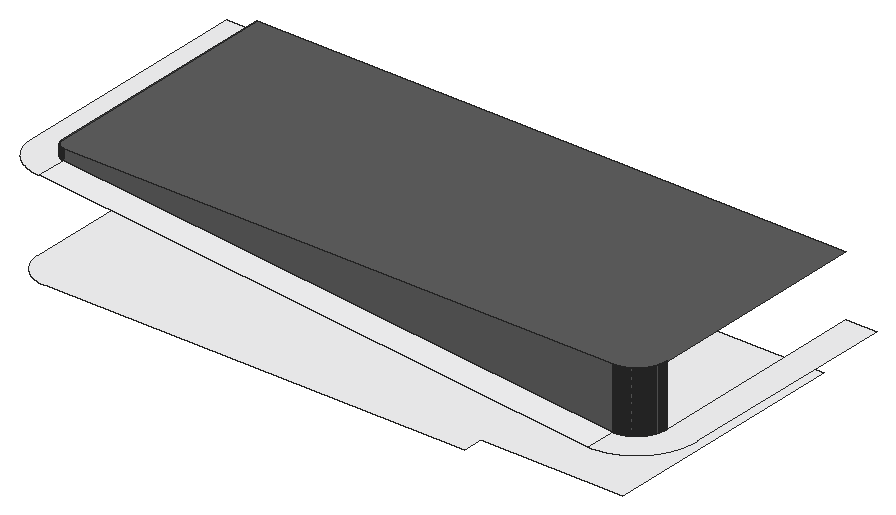
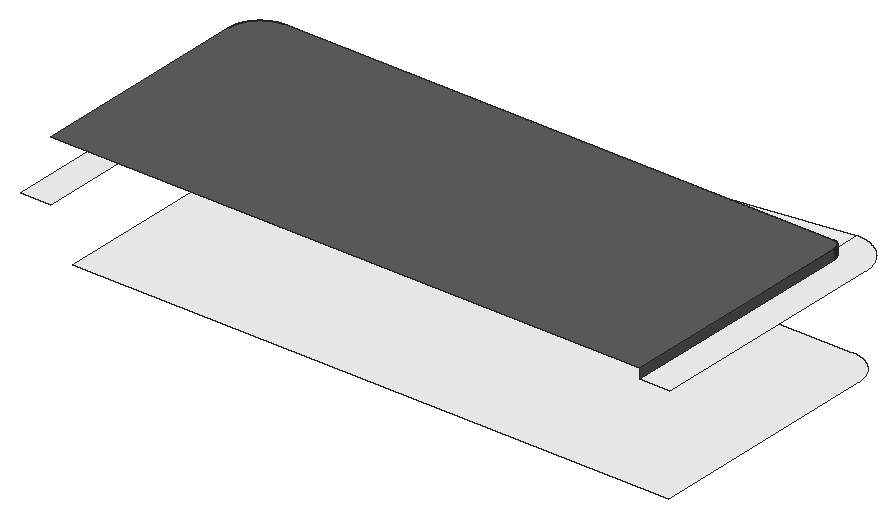
# SketchUp Ruby script. Lengths in inches.
U = 1.inch
M = Sketchup.active_model
def pt(a) = Geom::Point3d.new(a.map { |v| v * U })
def face(e, loops, mat)
  f = e.add_face(loops[0].map { |a| pt(a) })
  loops[1..].each { |l| e.add_face(l.map { |a| pt(a) }).erase! }
  f.material = f.back_material = mat if mat
  f
end
# faces: each face lists its corners as indices into pts; further lists are holes
def faces(e, pts, list, mat = nil) = list.each { |f| face(e, (f[0].is_a?(Array) ? f : [f]).map { |l| l.map { |i| pts[i] } }, mat) }
# xy, xz, yz: faces in a plane at the given z, y or x. An outline is a flat list of corners, or four numbers for a rectangle; further outlines are holes
def ring(l) = l.size == 4 ? [[l[0], l[1]], [l[2], l[1]], [l[2], l[3]], [l[0], l[3]]] : l.each_slice(2).to_a
def flat(e, list, mat, &to3) = list.each { |f| face(e, (f[0].is_a?(Array) ? f : [f]).map { |l| ring(l).map { |u, v| to3.(u, v) } }, mat) }
def xy(e, z, list, mat = nil) = flat(e, list, mat) { |x, y| [x, y, z] }
def xz(e, y, list, mat = nil) = flat(e, list, mat) { |x, z| [x, y, z] }
def yz(e, x, list, mat = nil) = flat(e, list, mat) { |y, z| [x, y, z] }
def lines(e, pts, list) = list.each { |a, b| e.add_line(pt(pts[a]), pt(pts[b])) }
# prism: a flat outline (further loops are holes) pulled along v
def prism(e, loops, v, mat = nil)
  f = face(e, loops, mat); d = Geom::Vector3d.new(v.map { |x| x * U })
  f.pushpull(f.normal.samedirection?(d) ? d.length : -d.length)
end
def box(e, o, s, mat = nil) = prism(e, [[o, [o[0] + s[0], o[1], o[2]], [o[0] + s[0], o[1] + s[1], o[2]], [o[0], o[1] + s[1], o[2]]]], [0, 0, s[2]], mat)
def at(x, y, z, deg = 0) = Geom::Transformation.translation(pt([x, y, z])) * Geom::Transformation.rotation(ORIGIN, Z_AXIS, deg.degrees)
def axes(o, x, y, z) = Geom::Transformation.new([*x, 0, *y, 0, *z, 0, *pt(o).to_a, 1])
def part(name) = M.definitions.add(name)
# library, detail: a bought-in or finely detailed component or shape, given as its bounding box
def library(name, o, s) = part(name).tap { |d| box(d.entities, o, s) }
def detail(e, o, s) = box(e.add_group.entities, o, s)
def put(e, d, t, mat = nil) = e.add_instance(d, t).tap { |i| i.material = mat if mat }
def group(e, t, mat = nil) = e.add_group.tap { |g| g.transformation = t; g.material = mat if mat }.entities
root = M.entities
M.materials.add("1421 AP 8232 ELEGANT GREY").color = [96, 96, 96]
M.materials.add("[Quartz Light Grey]").color = [251, 251, 252]
xy(root,234,[[47.74,189,47.61,189.01,47.48,189.01,47.22,189.03,47.08,189.04,46.95,189.05,46.69,189.09,46.57,189.1,46.4375,189.125,46.31,189.14,46.18,189.17,46.05,189.19,45.79,189.25,45.67,189.28,45.41,189.34,45.29,189.375,45.16,189.41,45.03,189.45,44.79,189.53,44.66,189.57,44.54,189.62,44.42,189.66,44.29,189.71,44.17,189.76,44.05,189.8125,43.93,189.86,43.8125,189.92,43.69,189.97,43.58,190.03,43.34,190.15,43.23,190.21,43.11,190.28,43,190.34,42.89,190.41,42.78,190.47,42.66,190.54,42.55,190.61,42.44,190.69,42.34,190.76,42.23,190.83,42.12,190.91,42.02,190.99,41.91,191.07,41.71,191.23,41.61,191.3125,41.51,191.4,41.41,191.48,41.21,191.66,41.12,191.75,41.02,191.84,40.84,192.02,40.75,192.12,40.66,192.21,40.48,192.41,40.4,192.51,40.3125,192.61,40.23,192.71,40.07,192.91,39.99,193.02,39.91,193.12,39.83,193.23,39.76,193.34,39.69,193.44,39.61,193.55,39.54,193.66,39.47,193.78,39.41,193.89,39.34,194,39.28,194.11,39.21,194.23,39.15,194.34,39.03,194.58,38.97,194.69,38.92,194.8125,38.86,194.93,38.8125,195.05,38.76,195.17,38.71,195.29,38.66,195.42,38.62,195.54,38.57,195.66,38.53,195.79,38.45,196.03,38.41,196.16,38.375,196.29,38.34,196.41,38.28,196.67,38.25,196.79,38.19,197.05,38.17,197.18,38.14,197.31,38.125,197.4375,38.1,197.57,38.09,197.69,38.05,197.95,38.04,198.08,38.03,198.22,38.01,198.48,38.01,198.61,38,198.74,38,269,214,269,214,195,172,195,172,189]],"[Quartz Light Grey]")
xy(root,249,[[210,187,210.24,187,210.47,187.01,210.71,187.01,210.94,187.02,211.18,187.04,211.41,187.06,211.65,187.08,211.88,187.1,212.12,187.125,212.35,187.15,212.58,187.1875,212.82,187.22,213.28,187.3,213.51,187.35,213.74,187.39,213.97,187.44,214.2,187.5,214.43,187.55,214.66,187.61,214.89,187.68,215.11,187.74,215.34,187.81,215.5625,187.88,215.79,187.96,216.01,188.03,216.23,188.11,216.45,188.2,216.67,188.28,217.11,188.46,217.32,188.56,217.54,188.65,217.75,188.75,217.96,188.86,218.17,188.96,218.59,189.18,218.8,189.3,219,189.41,219.4,189.65,219.61,189.78,219.8,189.9,220,190.03,220.2,190.17,220.39,190.3,220.58,190.4375,220.77,190.58,220.96,190.72,221.14,190.86,221.33,191.01,221.51,191.16,221.69,191.3125,221.87,191.47,222.04,191.625,222.22,191.78,222.39,191.94,222.56,192.11,222.73,192.27,222.89,192.44,223.06,192.61,223.22,192.78,223.375,192.96,223.53,193.13,223.6875,193.31,223.84,193.49,223.99,193.67,224.14,193.86,224.28,194.04,224.42,194.23,224.5625,194.42,224.7,194.61,224.83,194.8,224.97,195,225.1,195.2,225.22,195.39,225.35,195.6,225.59,196,225.7,196.2,225.82,196.41,226.04,196.83,226.14,197.04,226.25,197.25,226.35,197.46,226.44,197.68,226.54,197.89,226.72,198.33,226.8,198.55,226.89,198.77,226.97,198.99,227.04,199.21,227.12,199.4375,227.19,199.66,227.26,199.89,227.32,200.11,227.39,200.34,227.45,200.57,227.5,200.8,227.56,201.03,227.61,201.26,227.65,201.49,227.7,201.72,227.78,202.18,227.8125,202.42,227.85,202.65,227.875,202.88,227.9,203.12,227.92,203.35,227.94,203.59,227.96,203.82,227.98,204.06,227.99,204.29,227.99,204.53,228,204.76,228,271,219,271,219,204.76,218.99,204.65,218.99,204.53,218.97,204.29,218.96,204.18,218.95,204.06,218.9375,203.94,218.92,203.83,218.91,203.71,218.89,203.59,218.87,203.48,218.83,203.24,218.8,203.13,218.78,203.01,218.75,202.9,218.72,202.78,218.66,202.56,218.63,202.44,218.6,202.33,218.48,202,218.44,201.88,218.36,201.66,218.31,201.56,218.27,201.45,218.17,201.23,218.125,201.125,218.07,201.02,218.02,200.91,217.96,200.81,217.91,200.71,217.85,200.6,217.55,200.1,217.48,200,217.42,199.9,217.35,199.81,217.28,199.71,217.21,199.62,217.14,199.52,217.07,199.43,216.99,199.34,216.92,199.25,216.84,199.15,216.77,199.07,216.6875,198.98,216.61,198.89,216.53,198.8,216.45,198.72,216.36,198.64,216.28,198.55,216.2,198.47,216.11,198.39,216.02,198.3125,215.93,198.23,215.85,198.16,215.75,198.08,215.66,198.01,215.57,197.93,215.48,197.86,215.38,197.79,215.29,197.72,215.19,197.65,215.1,197.58,215,197.52,214.9,197.45,214.4,197.15,214.29,197.09,214.19,197.04,214.09,196.98,213.98,196.93,213.875,196.875,213.77,196.83,213.55,196.73,213.44,196.69,213.34,196.64,213.12,196.56,213,196.52,212.67,196.4,212.56,196.37,212.44,196.34,212.22,196.28,212.1,196.25,211.99,196.22,211.87,196.2,211.76,196.17,211.52,196.13,211.41,196.11,211.29,196.09,211.17,196.08,211.06,196.0625,210.94,196.05,210.82,196.04,210.71,196.03,210.47,196.01,210.35,196.01,210.24,196,210,196]],"[Quartz Light Grey]")
xy(root,264,[[47.6875,187,48,187,48,196,47.84,196,47.8,196.01,47.73,196.01,47.6875,196.02,47.65,196.02,47.61,196.03,47.57,196.03,47.53,196.04,47.49,196.04,47.41,196.06,47.375,196.07,47.34,196.07,47.22,196.1,47.1875,196.11,47.15,196.125,47.11,196.13,47.07,196.15,47.04,196.16,47,196.17,46.96,196.19,46.92,196.2,46.89,196.21,46.85,196.23,46.82,196.24,46.74,196.28,46.71,196.29,46.67,196.31,46.64,196.33,46.6,196.35,46.57,196.36,46.53,196.38,46.47,196.42,46.43,196.44,46.37,196.48,46.33,196.51,46.24,196.57,46.21,196.6,46.17,196.62,46.14,196.64,46.11,196.67,46.08,196.69,46.05,196.72,46.02,196.74,45.96,196.8,45.93,196.82,45.91,196.85,45.85,196.91,45.82,196.93,45.8,196.96,45.74,197.02,45.72,197.05,45.69,197.08,45.67,197.11,45.64,197.14,45.62,197.17,45.6,197.21,45.57,197.24,45.51,197.33,45.48,197.37,45.44,197.43,45.42,197.47,45.38,197.53,45.36,197.57,45.35,197.6,45.33,197.64,45.31,197.67,45.29,197.71,45.28,197.74,45.24,197.82,45.23,197.85,45.21,197.89,45.2,197.92,45.19,197.96,45.17,198,45.16,198.04,45.15,198.07,45.13,198.11,45.125,198.15,45.11,198.1875,45.1,198.22,45.07,198.34,45.07,198.375,45.06,198.41,45.04,198.49,45.04,198.53,45.03,198.57,45.03,198.61,45.02,198.65,45.02,198.6875,45.01,198.73,45.01,198.8,45,198.84,45,271,36,271,36,198.6875,36.01,198.53,36.02,198.37,36.03,198.22,36.05,197.9,36.07,197.75,36.08,197.59,36.1,197.43,36.125,197.28,36.15,197.12,36.17,196.97,36.2,196.8125,36.23,196.66,36.26,196.51,36.3,196.35,36.33,196.2,36.37,196.05,36.41,195.89,36.49,195.59,36.64,195.14,36.6875,194.99,36.74,194.85,36.8,194.7,36.85,194.55,36.91,194.41,36.97,194.26,37.04,194.12,37.1,193.98,37.17,193.83,37.45,193.27,37.53,193.14,37.61,193,37.6875,192.86,37.77,192.73,37.85,192.6,37.9375,192.46,38.02,192.33,38.2,192.07,38.29,191.95,38.38,191.82,38.48,191.69,38.58,191.57,38.67,191.45,38.77,191.33,38.98,191.09,39.08,190.97,39.1875,190.85,39.3,190.74,39.4,190.625,39.51,190.51,39.625,190.4,39.74,190.3,39.85,190.1875,39.97,190.08,40.09,189.98,40.33,189.77,40.45,189.67,40.57,189.58,40.69,189.48,40.82,189.38,40.95,189.29,41.07,189.2,41.33,189.02,41.46,188.9375,41.6,188.85,41.73,188.77,41.86,188.6875,42,188.61,42.14,188.53,42.27,188.45,42.83,188.17,42.98,188.1,43.12,188.04,43.26,187.97,43.41,187.91,43.55,187.85,43.7,187.8,43.85,187.74,43.99,187.6875,44.14,187.64,44.59,187.49,44.89,187.41,45.05,187.37,45.2,187.33,45.35,187.3,45.51,187.26,45.66,187.23,45.8125,187.2,45.97,187.17,46.12,187.15,46.28,187.125,46.43,187.1,46.59,187.08,46.75,187.07,46.9,187.05,47.22,187.03,47.37,187.02,47.53,187.01]],"[Quartz Light Grey]")
xy(root,267,[[47.84,196,210.24,196,210.35,196.01,210.47,196.01,210.71,196.03,210.82,196.04,210.94,196.05,211.06,196.0625,211.17,196.08,211.29,196.09,211.41,196.11,211.52,196.13,211.76,196.17,211.87,196.2,211.99,196.22,212.1,196.25,212.22,196.28,212.44,196.34,212.56,196.37,212.67,196.4,213,196.52,213.12,196.56,213.34,196.64,213.44,196.69,213.55,196.73,213.77,196.83,213.875,196.875,213.98,196.93,214.09,196.98,214.19,197.04,214.29,197.09,214.4,197.15,214.9,197.45,215,197.52,215.1,197.58,215.19,197.65,215.29,197.72,215.38,197.79,215.48,197.86,215.57,197.93,215.66,198.01,215.75,198.08,215.85,198.16,215.93,198.23,216.02,198.3125,216.11,198.39,216.2,198.47,216.28,198.55,216.36,198.64,216.45,198.72,216.53,198.8,216.61,198.89,216.6875,198.98,216.77,199.07,216.84,199.15,216.92,199.25,216.99,199.34,217.07,199.43,217.14,199.52,217.21,199.62,217.28,199.71,217.35,199.81,217.42,199.9,217.48,200,217.55,200.1,217.85,200.6,217.91,200.71,217.96,200.81,218.02,200.91,218.07,201.02,218.125,201.125,218.17,201.23,218.27,201.45,218.31,201.56,218.36,201.66,218.44,201.88,218.48,202,218.6,202.33,218.63,202.44,218.66,202.56,218.72,202.78,218.75,202.9,218.78,203.01,218.8,203.13,218.83,203.24,218.87,203.48,218.89,203.59,218.91,203.71,218.92,203.83,218.9375,203.94,218.95,204.06,218.96,204.18,218.97,204.29,218.99,204.53,218.99,204.65,219,204.76,219,271,45,271,45,198.84,45.01,198.8,45.01,198.73,45.02,198.6875,45.02,198.65,45.03,198.61,45.03,198.57,45.04,198.53,45.04,198.49,45.06,198.41,45.07,198.375,45.07,198.34,45.1,198.22,45.11,198.1875,45.125,198.15,45.13,198.11,45.15,198.07,45.16,198.04,45.17,198,45.19,197.96,45.2,197.92,45.21,197.89,45.23,197.85,45.24,197.82,45.28,197.74,45.29,197.71,45.31,197.67,45.33,197.64,45.35,197.6,45.36,197.57,45.38,197.53,45.42,197.47,45.44,197.43,45.48,197.37,45.51,197.33,45.57,197.24,45.6,197.21,45.62,197.17,45.64,197.14,45.67,197.11,45.69,197.08,45.72,197.05,45.74,197.02,45.8,196.96,45.82,196.93,45.85,196.91,45.91,196.85,45.93,196.82,45.96,196.8,46.02,196.74,46.05,196.72,46.08,196.69,46.11,196.67,46.14,196.64,46.17,196.62,46.21,196.6,46.24,196.57,46.33,196.51,46.37,196.48,46.43,196.44,46.47,196.42,46.53,196.38,46.57,196.36,46.6,196.35,46.64,196.33,46.67,196.31,46.71,196.29,46.74,196.28,46.82,196.24,46.85,196.23,46.89,196.21,46.92,196.2,46.96,196.19,47,196.17,47.04,196.16,47.07,196.15,47.11,196.13,47.15,196.125,47.1875,196.11,47.22,196.1,47.34,196.07,47.375,196.07,47.41,196.06,47.49,196.04,47.53,196.04,47.57,196.03,47.61,196.03,47.65,196.02,47.6875,196.02,47.73,196.01,47.8,196.01]],"1421 AP 8232 ELEGANT GREY")
xz(root,196,[[210,249,210,267,48,267,48,264],[210,249,210.12,267],[210.12,249,210.24,267],[47.84,264,47.88,267],[47.88,264,47.92,267],
  [47.92,264,47.96,267],[47.96,264,48,267]],"1421 AP 8232 ELEGANT GREY")
xz(root,196.01,[[210.35,249,210.47,267],[47.73,264,47.76,267],[47.76,264,47.8,267]],"1421 AP 8232 ELEGANT GREY")
xz(root,196.02,[[47.65,264,47.6875,267]],"1421 AP 8232 ELEGANT GREY")
xz(root,196.03,[[47.57,264,47.61,267]],"1421 AP 8232 ELEGANT GREY")
xz(root,196.04,[[47.49,264,47.53,267]],"1421 AP 8232 ELEGANT GREY")
xz(root,196.07,[[47.34,264,47.375,267]],"1421 AP 8232 ELEGANT GREY")
yz(root,45,[[198.84,264,198.88,267],[198.88,264,198.92,267],[198.92,264,198.96,267],[198.96,264,199,267],[199,264,271,267]],"1421 AP 8232 ELEGANT GREY")
yz(root,45.01,[[198.73,264,198.76,267],[198.76,264,198.8,267]],"1421 AP 8232 ELEGANT GREY")
yz(root,45.02,[[198.65,264,198.6875,267]],"1421 AP 8232 ELEGANT GREY")
yz(root,45.03,[[198.57,264,198.61,267]],"1421 AP 8232 ELEGANT GREY")
yz(root,45.04,[[198.49,264,198.53,267]],"1421 AP 8232 ELEGANT GREY")
yz(root,45.07,[[198.34,264,198.375,267]],"1421 AP 8232 ELEGANT GREY")
yz(root,218.99,[[204.53,249,204.65,267]],"1421 AP 8232 ELEGANT GREY")
yz(root,219,[[204.76,249,204.88,267],[204.88,249,205,267]],"1421 AP 8232 ELEGANT GREY")
p = [[48,187,264],[210,187,249],[210,196,249],[48,196,264],[210.35,196.01,249],[210.35,196.01,267],
  [210.24,196,267],[210.24,196,249],[210.59,196.02,249],[210.59,196.02,267],[210.47,196.01,267],[210.47,196.01,249],
  [210.71,196.03,249],[210.71,196.03,267],[210.82,196.04,249],[210.82,196.04,267],[210.94,196.05,249],[210.94,196.05,267],
  [211.06,196.0625,249],[211.06,196.0625,267],[211.17,196.08,249],[211.17,196.08,267],[211.29,196.09,249],[211.29,196.09,267],
  [211.41,196.11,249],[211.41,196.11,267],[211.52,196.13,249],[211.52,196.13,267],[211.64,196.15,249],[211.64,196.15,267],
  [211.76,196.17,249],[211.76,196.17,267],[211.87,196.2,249],[211.87,196.2,267],[211.99,196.22,249],[211.99,196.22,267],
  [212.1,196.25,249],[212.1,196.25,267],[212.22,196.28,249],[212.22,196.28,267],[212.33,196.31,249],[212.33,196.31,267],
  [212.44,196.34,249],[212.44,196.34,267],[212.56,196.37,249],[212.56,196.37,267],[212.67,196.4,249],[212.67,196.4,267],
  [212.78,196.44,249],[212.78,196.44,267],[212.89,196.48,249],[212.89,196.48,267],[213,196.52,249],[213,196.52,267],
  [213.12,196.56,249],[213.12,196.56,267],[213.23,196.6,249],[213.23,196.6,267],[213.34,196.64,249],[213.34,196.64,267],
  [213.44,196.69,249],[213.44,196.69,267],[213.55,196.73,249],[213.55,196.73,267],[213.66,196.78,249],[213.66,196.78,267],
  [213.77,196.83,249],[213.77,196.83,267],[213.875,196.875,249],[213.875,196.875,267],[213.98,196.93,249],[213.98,196.93,267],
  [214.09,196.98,249],[214.09,196.98,267],[214.19,197.04,249],[214.19,197.04,267],[214.29,197.09,249],[214.29,197.09,267],
  [214.4,197.15,249],[214.4,197.15,267],[214.5,197.21,249],[214.5,197.21,267],[214.6,197.27,249],[214.6,197.27,267],
  [214.7,197.33,249],[214.7,197.33,267],[214.8,197.39,249],[214.8,197.39,267],[214.9,197.45,249],[214.9,197.45,267],
  [215,197.52,249],[215,197.52,267],[215.1,197.58,249],[215.1,197.58,267],[215.19,197.65,249],[215.19,197.65,267],
  [215.29,197.72,249],[215.29,197.72,267],[215.38,197.79,249],[215.38,197.79,267],[215.48,197.86,249],[215.48,197.86,267],
  [215.57,197.93,249],[215.57,197.93,267],[215.66,198.01,249],[215.66,198.01,267],[215.75,198.08,249],[215.75,198.08,267],
  [215.85,198.16,249],[215.85,198.16,267],[215.93,198.23,249],[215.93,198.23,267],[216.02,198.3125,249],[216.02,198.3125,267],
  [216.11,198.39,249],[216.11,198.39,267],[216.2,198.47,249],[216.2,198.47,267],[216.28,198.55,249],[216.28,198.55,267],
  [216.36,198.64,249],[216.36,198.64,267],[216.45,198.72,249],[216.45,198.72,267],[216.53,198.8,249],[216.53,198.8,267],
  [216.61,198.89,249],[216.61,198.89,267],[216.6875,198.98,249],[216.6875,198.98,267],[216.77,199.07,249],[216.77,199.07,267],
  [216.84,199.15,249],[216.84,199.15,267],[216.92,199.25,249],[216.92,199.25,267],[216.99,199.34,249],[216.99,199.34,267],
  [217.07,199.43,249],[217.07,199.43,267],[217.14,199.52,249],[217.14,199.52,267],[217.21,199.62,249],[217.21,199.62,267],
  [217.28,199.71,249],[217.28,199.71,267],[217.35,199.81,249],[217.35,199.81,267],[217.42,199.9,249],[217.42,199.9,267],
  [217.48,200,249],[217.48,200,267],[217.55,200.1,249],[217.55,200.1,267],[217.61,200.2,249],[217.61,200.2,267],
  [217.67,200.3,249],[217.67,200.3,267],[217.73,200.4,249],[217.73,200.4,267],[217.79,200.5,249],[217.79,200.5,267],
  [217.85,200.6,249],[217.85,200.6,267],[217.91,200.71,249],[217.91,200.71,267],[217.96,200.81,249],[217.96,200.81,267],
  [218.02,200.91,249],[218.02,200.91,267],[218.07,201.02,249],[218.07,201.02,267],[218.125,201.125,249],[218.125,201.125,267],
  [218.17,201.23,249],[218.17,201.23,267],[218.22,201.34,249],[218.22,201.34,267],[218.27,201.45,249],[218.27,201.45,267],
  [218.31,201.56,249],[218.31,201.56,267],[218.36,201.66,249],[218.36,201.66,267],[218.4,201.77,249],[218.4,201.77,267],
  [218.44,201.88,249],[218.44,201.88,267],[218.48,202,249],[218.48,202,267],[218.52,202.11,249],[218.52,202.11,267],
  [218.56,202.22,249],[218.56,202.22,267],[218.6,202.33,249],[218.6,202.33,267],[218.63,202.44,249],[218.63,202.44,267],
  [218.66,202.56,249],[218.66,202.56,267],[218.69,202.67,249],[218.69,202.67,267],[218.72,202.78,249],[218.72,202.78,267],
  [218.75,202.9,249],[218.75,202.9,267],[218.78,203.01,249],[218.78,203.01,267],[218.8,203.13,249],[218.8,203.13,267],
  [218.83,203.24,249],[218.83,203.24,267],[218.85,203.36,249],[218.85,203.36,267],[218.87,203.48,249],[218.87,203.48,267],
  [218.89,203.59,249],[218.89,203.59,267],[218.91,203.71,249],[218.91,203.71,267],[218.92,203.83,249],[218.92,203.83,267],
  [218.9375,203.94,249],[218.9375,203.94,267],[218.95,204.06,249],[218.95,204.06,267],[218.96,204.18,249],[218.96,204.18,267],
  [218.97,204.29,249],[218.97,204.29,267],[218.98,204.41,249],[218.98,204.41,267],[218.99,204.53,249],[218.99,204.53,267],
  [219,204.76,249],[219,204.76,267],[218.99,204.65,267],[218.99,204.65,249],[47.53,196.04,264],[47.57,196.03,264],
  [47.57,196.03,267],[47.53,196.04,267],[47.45,196.05,264],[47.49,196.04,264],[47.49,196.04,267],[47.45,196.05,267],
  [47.61,196.03,264],[47.65,196.02,264],[47.65,196.02,267],[47.61,196.03,267],[47.6875,196.02,264],[47.73,196.01,264],
  [47.73,196.01,267],[47.6875,196.02,267],[47.8,196.01,264],[47.84,196,264],[47.84,196,267],[47.8,196.01,267],
  [47.04,196.16,264],[47.07,196.15,264],[47.07,196.15,267],[47.04,196.16,267],[47.15,196.125,264],[47.1875,196.11,264],
  [47.1875,196.11,267],[47.15,196.125,267],[47.11,196.13,264],[47.11,196.13,267],[47.22,196.1,264],[47.26,196.09,264],
  [47.26,196.09,267],[47.22,196.1,267],[47.3,196.08,264],[47.34,196.07,264],[47.34,196.07,267],[47.3,196.08,267],
  [47.41,196.06,264],[47.41,196.06,267],[47.375,196.07,264],[47.375,196.07,267],[46.82,196.24,264],[46.85,196.23,264],
  [46.85,196.23,267],[46.82,196.24,267],[46.78,196.26,264],[46.78,196.26,267],[46.92,196.2,264],[46.96,196.19,264],
  [46.96,196.19,267],[46.92,196.2,267],[46.89,196.21,264],[46.89,196.21,267],[47,196.17,264],[47,196.17,267],
  [46.64,196.33,264],[46.67,196.31,264],[46.67,196.31,267],[46.64,196.33,267],[46.6,196.35,264],[46.6,196.35,267],
  [46.57,196.36,264],[46.57,196.36,267],[46.74,196.28,264],[46.74,196.28,267],[46.71,196.29,264],[46.71,196.29,267],
  [46.43,196.44,264],[46.47,196.42,264],[46.47,196.42,267],[46.43,196.44,267],[46.4,196.46,264],[46.4,196.46,267],
  [46.53,196.38,264],[46.53,196.38,267],[46.5,196.4,264],[46.5,196.4,267],[46.33,196.51,264],[46.37,196.48,264],
  [46.37,196.48,267],[46.33,196.51,267],[46.3,196.53,264],[46.3,196.53,267],[46.27,196.55,264],[46.27,196.55,267],
  [46.14,196.64,264],[46.17,196.62,264],[46.17,196.62,267],[46.14,196.64,267],[46.11,196.67,264],[46.11,196.67,267],
  [46.24,196.57,264],[46.24,196.57,267],[46.21,196.6,264],[46.21,196.6,267],[46.02,196.74,264],[46.05,196.72,264],
  [46.05,196.72,267],[46.02,196.74,267],[45.99,196.77,264],[45.99,196.77,267],[46.08,196.69,264],[46.08,196.69,267],
  [45.93,196.82,264],[45.96,196.8,264],[45.96,196.8,267],[45.93,196.82,267],[45.91,196.85,264],[45.91,196.85,267],
  [45.82,196.93,264],[45.85,196.91,264],[45.85,196.91,267],[45.82,196.93,267],[45.8,196.96,264],[45.8,196.96,267],
  [45.88,196.88,264],[45.88,196.88,267],[45.74,197.02,264],[45.77,196.99,264],[45.77,196.99,267],[45.74,197.02,267],
  [45.72,197.05,264],[45.72,197.05,267],[45.64,197.14,264],[45.67,197.11,264],[45.67,197.11,267],[45.64,197.14,267],
  [45.62,197.17,264],[45.62,197.17,267],[45.69,197.08,264],[45.69,197.08,267],[45.6,197.21,264],[45.6,197.21,267],
  [45.57,197.24,264],[45.57,197.24,267],[45.55,197.27,264],[45.55,197.27,267],[45.53,197.3,264],[45.53,197.3,267],
  [45.51,197.33,264],[45.51,197.33,267],[45.48,197.37,264],[45.48,197.37,267],[45.44,197.43,264],[45.46,197.4,264],
  [45.46,197.4,267],[45.44,197.43,267],[45.42,197.47,264],[45.42,197.47,267],[45.4,197.5,264],[45.4,197.5,267],
  [45.38,197.53,264],[45.38,197.53,267],[45.36,197.57,264],[45.36,197.57,267],[45.35,197.6,264],[45.35,197.6,267],
  [45.33,197.64,264],[45.33,197.64,267],[45.31,197.67,264],[45.31,197.67,267],[45.29,197.71,264],[45.29,197.71,267],
  [45.28,197.74,264],[45.28,197.74,267],[45.26,197.78,264],[45.26,197.78,267],[45.24,197.82,264],[45.24,197.82,267],
  [45.23,197.85,264],[45.23,197.85,267],[45.21,197.89,264],[45.21,197.89,267],[45.2,197.92,264],[45.2,197.92,267],
  [45.19,197.96,264],[45.19,197.96,267],[45.15,198.07,264],[45.16,198.04,264],[45.16,198.04,267],[45.15,198.07,267],
  [45.17,198,264],[45.17,198,267],[45.13,198.11,264],[45.13,198.11,267],[45.125,198.15,264],[45.125,198.15,267],
  [45.11,198.1875,264],[45.11,198.1875,267],[45.1,198.22,264],[45.1,198.22,267],[45.09,198.26,264],[45.09,198.26,267],
  [45.08,198.3,264],[45.08,198.3,267],[45.07,198.34,264],[45.07,198.34,267],[45.06,198.41,264],[45.07,198.375,264],
  [45.07,198.375,267],[45.06,198.41,267],[45.05,198.45,264],[45.05,198.45,267],[45.04,198.49,264],[45.04,198.49,267],
  [45.03,198.57,264],[45.04,198.53,264],[45.04,198.53,267],[45.03,198.57,267],[45.02,198.65,264],[45.03,198.61,264],
  [45.03,198.61,267],[45.02,198.65,267],[45.01,198.73,264],[45.02,198.6875,264],[45.02,198.6875,267],[45.01,198.73,267],
  [45,198.84,264],[45.01,198.8,264],[45.01,198.8,267],[45,198.84,267]]
faces(root,p,[[0,1,2,3]],"[Quartz Light Grey]")
faces(root,p,[[4,5,6,7],[8,9,10,11],[12,13,9,8],[14,15,13,12],[16,17,15,14],[18,19,17,16],[20,21,19,18],[22,23,21,20],
  [24,25,23,22],[26,27,25,24],[28,29,27,26],[30,31,29,28],[32,33,31,30],[34,35,33,32],[36,37,35,34],[38,39,37,36],
  [40,41,39,38],[42,43,41,40],[44,45,43,42],[46,47,45,44],[48,49,47,46],[50,51,49,48],[52,53,51,50],[54,55,53,52],
  [56,57,55,54],[58,59,57,56],[60,61,59,58],[62,63,61,60],[64,65,63,62],[66,67,65,64],[68,69,67,66],[70,71,69,68],
  [72,73,71,70],[74,75,73,72],[76,77,75,74],[78,79,77,76],[80,81,79,78],[82,83,81,80],[84,85,83,82],[86,87,85,84],
  [88,89,87,86],[90,91,89,88],[92,93,91,90],[94,95,93,92],[96,97,95,94],[98,99,97,96],[100,101,99,98],[102,103,101,100],
  [104,105,103,102],[106,107,105,104],[108,109,107,106],[110,111,109,108],[112,113,111,110],[114,115,113,112],[116,117,115,114],[118,119,117,116],
  [120,121,119,118],[122,123,121,120],[124,125,123,122],[126,127,125,124],[128,129,127,126],[130,131,129,128],[132,133,131,130],[134,135,133,132],
  [136,137,135,134],[138,139,137,136],[140,141,139,138],[142,143,141,140],[144,145,143,142],[146,147,145,144],[148,149,147,146],[150,151,149,148],
  [152,153,151,150],[154,155,153,152],[156,157,155,154],[158,159,157,156],[160,161,159,158],[162,163,161,160],[164,165,163,162],[166,167,165,164],
  [168,169,167,166],[170,171,169,168],[172,173,171,170],[174,175,173,172],[176,177,175,174],[178,179,177,176],[180,181,179,178],[182,183,181,180],
  [184,185,183,182],[186,187,185,184],[188,189,187,186],[190,191,189,188],[192,193,191,190],[194,195,193,192],[196,197,195,194],[198,199,197,196],
  [200,201,199,198],[202,203,201,200],[204,205,203,202],[206,207,205,204],[208,209,207,206],[210,211,209,208],[212,213,211,210],[214,215,213,212],
  [216,217,215,214],[218,219,217,216],[220,221,219,218],[222,223,221,220],[224,225,223,222],[226,227,225,224],[228,229,227,226],[230,231,229,228],
  [232,233,231,230],[234,235,236,237],[238,239,240,241],[242,243,244,245],[246,247,248,249],[250,251,252,253],[254,255,256,257],[258,259,260,261],
  [262,263,264,265],[266,262,265,267],[259,266,267,260],[268,269,270,271],[263,268,271,264],[272,273,274,275],[269,272,275,270],[276,242,245,277],
  [278,276,277,279],[280,281,282,283],[284,280,283,285],[286,287,288,289],[290,286,289,291],[281,290,291,282],[292,258,261,293],[287,292,293,288],
  [294,295,296,297],[298,294,297,299],[300,298,299,301],[302,284,285,303],[304,302,303,305],[295,304,305,296],[306,307,308,309],[310,306,309,311],
  [312,300,301,313],[314,312,313,315],[307,314,315,308],[316,317,318,319],[320,316,319,321],[322,320,321,323],[317,310,311,318],[324,325,326,327],
  [328,324,327,329],[330,322,323,331],[332,330,331,333],[325,332,333,326],[334,335,336,337],[338,334,337,339],[340,328,329,341],[335,340,341,336],
  [342,343,344,345],[346,342,345,347],[343,338,339,344],[348,349,350,351],[352,348,351,353],[354,346,347,355],[349,354,355,350],[356,357,358,359],
  [360,356,359,361],[357,352,353,358],[362,363,364,365],[366,362,365,367],[368,360,361,369],[363,368,369,364],[370,366,367,371],[372,370,371,373],
  [374,372,373,375],[376,374,375,377],[378,376,377,379],[380,378,379,381],[382,383,384,385],[386,382,385,387],[383,380,381,384],[388,386,387,389],
  [390,388,389,391],[392,390,391,393],[394,392,393,395],[396,394,395,397],[398,396,397,399],[400,398,399,401],[402,400,401,403],[404,402,403,405],
  [406,404,405,407],[408,406,407,409],[410,408,409,411],[412,410,411,413],[414,412,413,415],[416,417,418,419],[420,414,415,421],[417,420,421,418],
  [422,416,419,423],[424,422,423,425],[426,424,425,427],[428,426,427,429],[430,428,429,431],[432,430,431,433],[434,432,433,435],[436,437,438,439],
  [440,436,439,441],[442,440,441,443],[444,445,446,447],[448,449,450,451],[452,453,454,455],[456,457,458,459]],"1421 AP 8232 ELEGANT GREY")
